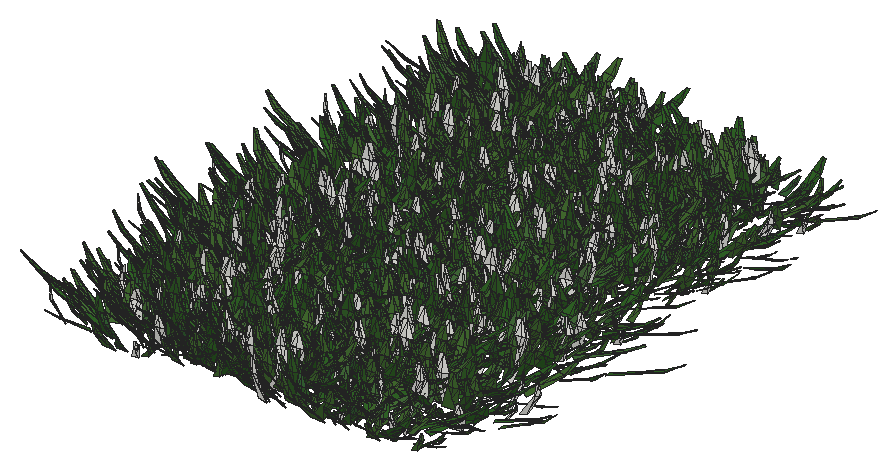
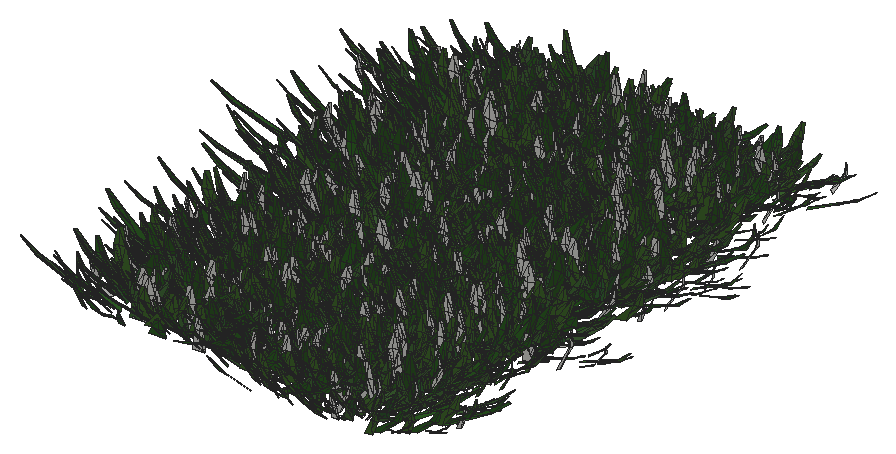
# SketchUp Ruby script. Lengths in inches.
U = 1.inch
M = Sketchup.active_model
def pt(a) = Geom::Point3d.new(a.map { |v| v * U })
def face(e, loops, mat)
  f = e.add_face(loops[0].map { |a| pt(a) })
  loops[1..].each { |l| e.add_face(l.map { |a| pt(a) }).erase! }
  f.material = f.back_material = mat if mat
  f
end
# faces: each face lists its corners as indices into pts; further lists are holes
def faces(e, pts, list, mat = nil) = list.each { |f| face(e, (f[0].is_a?(Array) ? f : [f]).map { |l| l.map { |i| pts[i] } }, mat) }
# xy, xz, yz: faces in a plane at the given z, y or x. An outline is a flat list of corners, or four numbers for a rectangle; further outlines are holes
def ring(l) = l.size == 4 ? [[l[0], l[1]], [l[2], l[1]], [l[2], l[3]], [l[0], l[3]]] : l.each_slice(2).to_a
def flat(e, list, mat, &to3) = list.each { |f| face(e, (f[0].is_a?(Array) ? f : [f]).map { |l| ring(l).map { |u, v| to3.(u, v) } }, mat) }
def xy(e, z, list, mat = nil) = flat(e, list, mat) { |x, y| [x, y, z] }
def xz(e, y, list, mat = nil) = flat(e, list, mat) { |x, z| [x, y, z] }
def yz(e, x, list, mat = nil) = flat(e, list, mat) { |y, z| [x, y, z] }
def lines(e, pts, list) = list.each { |a, b| e.add_line(pt(pts[a]), pt(pts[b])) }
# prism: a flat outline (further loops are holes) pulled along v
def prism(e, loops, v, mat = nil)
  f = face(e, loops, mat); d = Geom::Vector3d.new(v.map { |x| x * U })
  f.pushpull(f.normal.samedirection?(d) ? d.length : -d.length)
end
def box(e, o, s, mat = nil) = prism(e, [[o, [o[0] + s[0], o[1], o[2]], [o[0] + s[0], o[1] + s[1], o[2]], [o[0], o[1] + s[1], o[2]]]], [0, 0, s[2]], mat)
def at(x, y, z, deg = 0) = Geom::Transformation.translation(pt([x, y, z])) * Geom::Transformation.rotation(ORIGIN, Z_AXIS, deg.degrees)
def axes(o, x, y, z) = Geom::Transformation.new([*x, 0, *y, 0, *z, 0, *pt(o).to_a, 1])
def part(name) = M.definitions.add(name)
# library, detail: a bought-in or finely detailed component or shape, given as its bounding box
def library(name, o, s) = part(name).tap { |d| box(d.entities, o, s) }
def detail(e, o, s) = box(e.add_group.entities, o, s)
def put(e, d, t, mat = nil) = e.add_instance(d, t).tap { |i| i.material = mat if mat }
def group(e, t, mat = nil) = e.add_group.tap { |g| g.transformation = t; g.material = mat if mat }.entities
root = M.entities
M.materials.add("Material82").color = [68, 110, 58]
M.materials.add("Material83").color = [48, 90, 38]
M.materials.add("Material84").color = [68, 110, 48]
M.materials.add("Material85").color = [48, 90, 48]
M.materials.add("Material86").color = [58, 110, 58]
M.materials.add("Material87").color = [58, 90, 38]
M.materials.add("Material88").color = [68, 100, 58]
M.materials.add("Material89").color = [48, 100, 38]
c1 = part("grass00")
p = [[-0.6875,0.15,0],[-0.56,0.08,5.52],[-0.04,0.03,2.76],[0.48,-0.02,0],[0.35,-0.02,5.52],[-0.1,-0.14,5.52],
  [-0.12,0.65,8.37],[-0.42,0.65,8.37]]
faces(c1.entities,p,[[0,1,2,3],[3,2,4],[1,5,2],[5,4,2],[1,6,5],[4,5,6],[7,6,1]])
c2 = part("Group16\#1")
put(c2.entities,c1,axes([1.44,-0.61,-0.01],[0.05352,0.12609,0],[-0.10704,0.04543,0.07239],[0.06664,-0.02828,0.11628]),"Material85")
put(c2.entities,c1,axes([0.76,-0.15,-0.01],[0.04676,0.24062,0],[-0.23162,0.04501,0.06642],[0.0652,-0.01267,0.23595]),"Material82")
put(c2.entities,c1,axes([0.79,0.01,-0.01],[-0.00606,0.34651,0],[-0.34381,-0.00602,0.0432],[0.04319,0.00076,0.34386]))
put(c2.entities,c1,axes([1,0.23,-0.01],[-0.07192,0.31144,0],[-0.28722,-0.06632,0.1236],[0.12043,0.02781,0.29478]),"Material84")
put(c2.entities,c1,axes([1.66,0.77,-0.01],[-0.13828,0.29651,0],[-0.21551,-0.1005,0.22471],[0.20365,0.09498,0.23779]),"Material89")
put(c2.entities,c1,axes([0.6875,0.52,-0.01],[-0.18126,0.24051,0],[-0.22746,-0.17142,0.09788],[0.07817,0.05891,0.28481]),"Material84")
put(c2.entities,c1,axes([0.68,0.78,-0.01],[-0.215,0.18688,0],[-0.12385,-0.14248,0.21334],[0.13995,0.16101,0.18878]),"Material82")
put(c2.entities,c1,axes([0.56,1,-0.01],[-0.13756,0.07624,0],[-0.06159,-0.11112,0.0927],[0.04494,0.08108,0.12705]),"Material84")
put(c2.entities,c1,axes([0.2,0.64,-0.01],[-0.23729,0.07254,0],[-0.05711,-0.18681,0.153],[0.04473,0.14632,0.19535]),"Material89")
put(c2.entities,c1,axes([0.0625,0.72,-0.01],[-0.28874,0.02525,0],[-0.02179,-0.24916,0.14647],[0.01276,0.14591,0.25012]),"Material82")
put(c2.entities,c1,axes([-0.08,0.62,-0.01],[-0.34089,-0.04187,0],[0.03255,-0.26504,0.216],[-0.02633,0.21439,0.26703]),"Material89")
put(c2.entities,c1,axes([-0.34,0.98,-0.01],[-0.14314,-0.0493,0],[0.04397,-0.12769,0.06843],[-0.02228,0.0647,0.13505]),"Material89")
put(c2.entities,c1,axes([-0.87,1.45,-0.01],[-0.23488,-0.14114,0],[0.13761,-0.22901,0.06087],[-0.03135,0.05217,0.26717]))
put(c2.entities,c1,axes([-0.72,0.77,-0.01],[-0.14208,-0.13251,0],[0.07209,-0.0773,0.16301],[-0.11118,0.11922,0.1057]),"Material89")
put(c2.entities,c1,axes([-0.62,0.43,-0.01],[-0.14845,-0.21203,0],[0.18654,-0.13061,0.12304],[-0.10079,0.07057,0.22772]),"Material82")
put(c2.entities,c1,axes([-0.68,0.29,-0.01],[-0.13639,-0.32136,0],[0.31723,-0.13464,0.05579],[-0.05136,0.0218,0.34462]),"Material83")
put(c2.entities,c1,axes([-0.64,0.125,-0.01],[-0.0458,-0.23569,0],[0.22124,-0.043,0.08276],[-0.08124,0.01579,0.22538]),"Material86")
put(c2.entities,c1,axes([-1.6,-0.03,-0.01],[0.00576,-0.32897,0],[0.27526,0.00482,0.18018],[-0.18015,-0.00315,0.2753]),"Material84")
put(c2.entities,c1,axes([-1.36,-0.31,-0.01],[0.05718,-0.24765,0],[0.18172,0.04196,0.17267],[-0.16825,-0.03885,0.1865]),"Material89")
put(c2.entities,c1,axes([-1.54,-0.72,-0.01],[0.06537,-0.14017,0],[0.13555,0.06321,0.03939],[-0.0357,-0.01665,0.14956]))
put(c2.entities,c1,axes([-1.19,-0.9,-0.01],[0.09597,-0.12735,0],[0.11214,0.08451,0.07557],[-0.06035,-0.04548,0.14042]),"Material88")
put(c2.entities,c1,axes([-0.47,-0.54,-0.01],[0.11588,-0.10072,0],[0.0618,0.0711,0.12124],[-0.07953,-0.0915,0.0942]))
put(c2.entities,c1,axes([-0.47,-0.84,-0.01],[0.11927,-0.0661,0],[0.06603,0.11913,0.00646],[-0.00313,-0.00565,0.13621]),"Material84")
put(c2.entities,c1,axes([-0.38,-1.24,-0.01],[0.28037,-0.08571,0],[0.0618,0.20215,0.20315],[-0.05939,-0.19428,0.21139]),"Material88")
put(c2.entities,c1,axes([-0.06,-0.66,-0.01],[0.22719,-0.01987,0],[0.01247,0.14255,0.17758],[-0.01547,-0.17691,0.1431]),"Material87")
put(c2.entities,c1,axes([0.11,-0.89,-0.01],[0.14882,0.01828,0],[-0.01058,0.08611,0.12229],[0.01491,-0.12138,0.08676]),"Material85")
put(c2.entities,c1,axes([0.25,-0.72,-0.01],[0.20481,0.07053,0],[-0.06206,0.18022,0.10291],[0.03351,-0.0973,0.1906]),"Material85")
put(c2.entities,c1,axes([0.85,-1.42,-0.01],[0.16481,0.09904,0],[-0.09472,0.15762,0.05616],[0.02893,-0.04814,0.18389]),"Material84")
put(c2.entities,c1,axes([1.01,-1.09,-0.01],[0.21858,0.20385,0],[-0.17495,0.1876,0.15339],[0.10462,-0.11218,0.25652]),"Material89")
put(c2.entities,c1,axes([1.01,-0.71,-0.01],[0.08733,0.12473,0],[-0.06445,0.04512,0.13037],[0.1068,-0.07477,0.07867]),"Material85")
c3 = part("Group15\#1")
put(c3.entities,c2,at(0,0,0))
c4 = part("3darcstudiotree_grass00\#1")
put(c4.entities,c3,at(0,0,0))
put(root,c4,axes([1703.49,1033.95,-29.74],[4.10302,-0.30694,0],[0.8385,1.74326,-0.00778],[0.00611,0.0127,1.42033]))
put(root,c4,axes([1703.88,1017.02,-29.74],[-2.0309,1.41107,0],[-3.96455,-0.88745,-0.03094],[-0.10652,-0.02384,1.35284]))
put(root,c4,axes([1703.7,1018.32,-29.74],[3.97679,-0.10087,0],[0.2922,1.7917,-0.04097],[0.01281,0.07857,1.66267]))
put(root,c4,axes([1704.37,1024.5,-29.74],[2.96266,-0.9536,0],[2.21709,1.07131,-0.03627],[0.16479,0.07963,1.88825]))
put(root,c4,axes([1705.53,1009.61,-29.74],[-2.64678,-1.36079,0],[3.05956,-0.92555,-0.03114],[0.16031,-0.04849,1.87535]))
put(root,c4,axes([1704.94,1048.64,-29.74],[2.77032,-1.11765,0],[2.79461,1.07735,-0.00015],[0.00071,0.00027,1.98495]))
put(root,c4,axes([1704.06,1012.55,-29.74],[1.36747,1.27936,0],[-3.91602,0.651,-0.04214],[-0.23603,0.03924,1.93625]))
put(root,c4,axes([1705.93,1031.41,-29.74],[-0.46652,-1.63259,0],[3.80254,-0.169,-0.02839],[0.12966,-0.00576,1.31807]))
put(root,c4,axes([1706.04,1038.09,-29.74],[-2.24585,-1.17679,0],[2.75058,-0.81643,-0.02546],[0.1532,-0.04547,1.94365]))
put(root,c4,axes([1706.63,1047.5,-29.74],[-3.1613,-1.38915,0],[3.20855,-1.13563,-0.02493],[0.08224,-0.02911,1.43253]))
put(root,c4,axes([1706.375,1051.55,-29.74],[-4.11217,-0.39094,0],[0.86082,-1.40827,-0.01967],[0.02693,-0.04406,1.60841]))
put(root,c4,axes([1705.74,1021.11,-29.74],[-2.52022,1.35688,0],[-2.71694,-0.78485,-0.02032],[-0.10759,-0.03108,1.65635]))
put(root,c4,axes([1706.38,1001.24,-29.74],[-3.93546,0.24929,0],[-0.63824,-1.56709,-0.04907],[-0.04216,-0.10352,1.63442]))
put(root,c4,axes([1705.97,1040.7,-29.74],[1.48309,-1.18944,0],[3.17184,0.61511,-0.04022],[0.27217,0.05278,1.99791]))
put(root,c4,axes([1705.13,998.44,-29.74],[-0.1961,1.67231,0],[-3.9427,-0.07191,-0.00948],[-0.04368,-0.0008,1.36423]))
put(root,c4,axes([1706.89,1042.42,-29.74],[-1.75334,-1.53625,0],[3.78301,-0.67151,-0.04331],[0.23983,-0.04257,1.88835]))
put(root,c4,axes([1707.03,1045.07,-29.74],[-1.47837,-1.71881,0],[3.4357,-0.4596,-0.01224],[0.08437,-0.01129,1.97883]))
put(root,c4,axes([1705.26,1022.94,-29.74],[0.89151,1.73156,0],[-4.53511,0.36315,-0.02679],[-0.1364,0.01092,1.80175]))
put(root,c4,axes([1705.84,1002.9,-29.74],[3.29656,-0.16392,0],[0.52833,1.6525,-0.05027],[0.03097,0.09687,1.55905]))
put(root,c4,axes([1705.26,1035.78,-29.74],[1.8424,1.14237,0],[-3.65624,0.91712,-0.00074],[-0.00371,0.00093,1.93092]))
put(root,c4,axes([1706.68,1014.64,-29.74],[2.92684,-0.73502,0],[1.91435,1.18558,-0.0345],[0.12831,0.07947,1.8497]))
put(root,c4,axes([1706.88,1005.96,-29.74],[0.10092,1.39888,0],[-4.08431,0.04583,-0.02239],[-0.13434,0.00151,1.83839]))
put(root,c4,axes([1706.96,1029.15,-29.74],[-0.46714,1.44095,0],[-4.49775,-0.22678,-0.0277],[-0.15196,-0.00766,1.87956]))
put(root,c4,axes([1708.99,1019.2,-29.74],[-2.63576,-1.28026,0],[3.53005,-1.13032,-0.02494],[0.11128,-0.03563,1.95866]))
put(root,c4,axes([1708.95,1053.33,-29.74],[-3.99047,-0.40873,0],[1.06863,-1.62266,-0.00758],[0.01027,-0.0156,1.7185]))
put(root,c4,axes([1708.68,1029.42,-29.74],[-0.06008,-1.38054,0],[4.09358,-0.02771,-0.0405],[0.24938,-0.00169,1.89003]))
put(root,c4,axes([1709.07,1036.51,-29.74],[-1.38876,-1.54798,0],[3.56891,-0.49797,-0.03351],[0.18812,-0.02625,1.68972]))
put(root,c4,axes([1709.6875,1046.76,-29.74],[-0.94917,-1.78727,0],[4.28932,-0.35429,-0.02019],[0.10216,-0.00844,1.69814]))
put(root,c4,axes([1709.52,1052.08,-29.74],[-0.90047,-1.75818,0],[4.05941,-0.32336,-0.03802],[0.21461,-0.0171,1.78771]))
put(root,c4,axes([1709.85,1021.48,-29.74],[-2.86404,-0.64452,0],[1.81455,-1.25407,-0.04344],[0.15373,-0.10625,1.9596]))
put(root,c4,axes([1710.09,1009.37,-29.74],[-1.66133,-1.5225,0],[4.09169,-0.6944,-0.04688],[0.21591,-0.03664,1.67419]))
put(root,c4,axes([1710.02,1015.88,-29.74],[-3.61877,0.99301,0],[-2.17277,-1.23149,-0.01001],[-0.02667,-0.01512,1.32974]))
put(root,c4,axes([1711.03,1027.38,-29.74],[-0.34586,-1.45501,0],[4.09876,-0.15153,-0.00863],[0.04038,-0.00149,1.44957]))
put(root,c4,axes([1711.61,1014.23,-29.74],[-1.55676,-1.64059,0],[4.33421,-0.63965,-0.05081],[0.20494,-0.03024,1.49393]))
put(root,c4,axes([1710.2,1024.86,-29.74],[4.37611,-0.60729,0],[1.31361,1.47222,-0.0057],[0.0109,0.01221,1.70987]))
put(root,c4,axes([1711.69,1042.79,-29.74],[-0.47275,-1.4969,0],[4.46074,-0.21911,-0.06365],[0.35527,-0.01745,1.89522]))
put(root,c4,axes([1711.28,1038.82,-29.74],[2.20658,-1.37183,0],[2.86337,0.71632,-0.01781],[0.08885,0.02223,1.50117]))
put(root,c4,axes([1710.93,1049.89,-29.74],[3.60935,-0.56815,0],[1.37625,1.35979,-0.02611],[0.05001,0.04941,1.43783]))
put(root,c4,axes([1712.11,1002.8,-29.74],[-3.927,-0.17218,0],[0.45946,-1.62986,-0.05312],[0.03146,-0.11159,1.67036]))
put(root,c4,axes([1711.02,1000.79,-29.74],[4.2823,-0.66393,0],[1.32307,1.32724,-0.00849],[0.02062,0.02068,1.79934]))
put(root,c4,axes([1712.3,1033.72,-29.74],[0.52677,-1.54843,0],[3.37532,0.17859,-0.00096],[0.0064,0.00034,1.71349]))
put(root,c4,axes([1712.28,1031.74,-29.74],[-3.78642,0.03695,0],[-0.11198,-1.78455,-0.01248],[-0.00125,-0.01991,1.37214]))
put(root,c4,axes([1712.5,1045.21,-29.74],[-3.50363,0.54877,0],[-1.37004,-1.36042,-0.04199],[-0.09387,-0.09321,1.68502]))
put(root,c4,axes([1712.33,1023.08,-29.74],[-3.78815,1.05417,0],[-2.08305,-1.1642,0],[-0.00001,-0.00001,1.91868]))
put(root,c4,axes([1711.59,999.37,-29.74],[3.14187,0.39177,0],[-1.17778,1.46906,-0.04459],[-0.07661,0.09555,1.66873]))
put(root,c4,axes([1712.79,1040.2,-29.74],[-4.05008,0.95977,0],[-1.76425,-1.15789,-0.02116],[-0.06339,-0.0416,1.49339]))
put(root,c4,axes([1712.49,1005.88,-29.74],[-2.14427,1.00131,0],[-3.09998,-1.03248,-0.03207],[-0.1604,-0.05342,1.99077]))
put(root,c4,axes([1712.68,1007.9,-29.74],[-3.03453,1.36043,0],[-3.50876,-1.21725,-0.06393],[-0.1925,-0.06678,1.40472]))
put(root,c4,axes([1712.5,1011.48,-29.74],[4.55933,-0.17295,0],[0.45061,1.84755,-0.06081],[0.02387,0.09789,1.44654]))
put(root,c4,axes([1714.37,1026.73,-29.74],[-0.03672,-1.35909,0],[4.67682,-0.01965,-0.05216],[0.20276,-0.00085,1.36288]))
put(root,c4,axes([1714.47,1012.2,-29.74],[0.13892,-1.80916,0],[4.0915,0.04886,-0.01983],[0.09749,0.00116,1.50947]))
put(root,c4,axes([1714.72,1045.11,-29.74],[-0.70107,-1.67232,0],[4.13597,-0.26967,-0.0168],[0.0818,-0.00533,1.55067]))
put(root,c4,axes([1714.86,1016.1875,-29.74],[-3.75519,-1.14447,0],[2.68213,-1.36874,-0.06061],[0.1619,-0.08262,1.43628]))
put(root,c4,axes([1714.39,1028.91,-29.74],[-0.54027,-1.6401,0],[3.32557,-0.17038,-0.04034],[0.23473,-0.01203,1.47504]))
put(root,c4,axes([1714.625,1024.72,-29.74],[-3.58356,0.46021,0],[-1.0679,-1.2933,-0.04555],[-0.08783,-0.10637,1.60995]))
put(root,c4,axes([1715.09,1002.92,-29.74],[-3.8661,0.57248,0],[-1.34665,-1.41442,-0.01194],[-0.02505,-0.02631,1.71307]))
put(root,c4,axes([1715.29,1010.36,-29.74],[-3.59396,1.08002,0],[-2.30452,-1.19271,-0.04347],[-0.15376,-0.07958,1.66314]))
put(root,c4,axes([1716.07,999.57,-29.74],[-3.24117,-0.71309,0],[1.62667,-1.14993,-0.00653],[0.01841,-0.01301,1.4475]))
put(root,c4,axes([1716.42,1043.23,-29.74],[-3.07387,-1.37226,0],[2.57369,-0.89663,-0.00245],[0.01347,-0.00469,1.8862]))
put(root,c4,axes([1714.6875,1049.15,-29.74],[0.39811,1.50692,0],[-3.94981,0.16229,-0.02993],[-0.16157,0.00664,1.61572]))
put(root,c4,axes([1714.78,1022.58,-29.74],[-0.46786,1.28327,0],[-3.81344,-0.21623,-0.00494],[-0.02392,-0.00136,1.4129]))
put(root,c4,axes([1716.57,1005.55,-29.74],[0.52643,-1.67667,0],[4.29673,0.20982,-0.00236],[0.01155,0.00056,1.5989]))
put(root,c4,axes([1715.29,1046.66,-29.74],[3.86987,-0.34459,0],[0.79622,1.39073,-0.03599],[0.03867,0.06754,1.32194]))
put(root,c4,axes([1716.37,1031.85,-29.74],[-3.89357,0.61481,0],[-1.50479,-1.48217,-0.00598],[-0.01246,-0.01228,1.70205]))
put(root,c4,axes([1715.52,1007.16,-29.74],[4.26757,-0.1267,0],[0.26808,1.40432,-0.02417],[0.01226,0.06424,1.80918]))
put(root,c4,axes([1715.57,1050.8125,-29.74],[0.18137,1.61713,0],[-3.86456,0.06741,-0.03464],[-0.18684,0.00326,1.56527]))
put(root,c4,axes([1715.35,1052.95,-29.74],[2.68425,0.98126,0],[-3.08103,1.31083,-0.0132],[-0.04194,0.01784,1.58767]))
put(root,c4,axes([1717.13,1018.3,-29.74],[-4.03193,0.12785,0],[-0.33897,-1.66251,-0.04274],[-0.01416,-0.06944,1.31001]))
put(root,c4,axes([1717.47,1033.54,-29.74],[-2.54975,-1.13663,0],[2.74994,-0.95943,-0.02762],[0.1264,-0.0441,1.68176]))
put(root,c4,axes([1715.75,1020.33,-29.74],[2.51292,1.08795,0],[-3.26468,1.1728,-0.05824],[-0.20485,0.07359,1.57486]))
put(root,c4,axes([1716.92,1037.86,-29.74],[2.12492,-1.52639,0],[3.32667,0.72027,-0.02765],[0.13101,0.02837,1.53783]))
put(root,c4,axes([1716.25,1001.04,-29.74],[2.57949,0.81299,0],[-2.19489,1.0831,-0.04441],[-0.18645,0.09201,1.772]))
put(root,c4,axes([1717.17,1040.1,-29.74],[2.26224,-1.2031,0],[3.43735,1.00525,-0.03781],[0.13632,0.03987,1.4396]))
put(root,c4,axes([1716.34,1035.7,-29.74],[0.64746,1.71828,0],[-3.59,0.21039,-0.03328],[-0.18561,0.01088,1.53387]))
put(root,c4,axes([1717.41,1013.91,-29.74],[1.65411,1.32331,0],[-4.02119,0.78176,-0.01549],[-0.05875,0.01142,1.42146]))
put(root,c4,axes([1720.15,1000.57,-29.74],[-1.99996,-1.21087,0],[3.64955,-0.93751,-0.00487],[0.02184,-0.00561,1.74651]))
put(root,c4,axes([1719.93,1049.92,-29.74],[-4.08637,0.5893,0],[-1.1512,-1.24155,-0.04181],[-0.0785,-0.08466,1.37365]))
put(root,c4,axes([1720.2,1033.33,-29.74],[0.94723,-1.59052,0],[4.2139,0.39031,-0.04288],[0.2193,0.02031,1.70449]))
put(root,c4,axes([1720.4,1003.34,-29.74],[0.76825,-1.34447,0],[4.07723,0.36235,-0.02216],[0.10533,0.00936,1.52603]))
put(root,c4,axes([1721.03,1039.85,-29.74],[-4.28344,0.1007,0],[-0.25434,-1.68266,-0.00226],[-0.00079,-0.00521,1.87745]))
put(root,c4,axes([1720.7,1044.92,-29.74],[1.6756,-1.36696,0],[3.5262,0.67226,-0.03335],[0.16368,0.0312,1.60043]))
put(root,c4,axes([1721.32,1012.25,-29.74],[-0.47602,-1.5827,0],[4.1601,-0.1946,-0.02638],[0.12052,-0.00564,1.44452]))
put(root,c4,axes([1720.36,1036.29,-29.74],[4.15464,-0.59094,0],[1.53872,1.68251,-0.06016],[0.09162,0.10018,1.52593]))
put(root,c4,axes([1720.62,1020.84,-29.74],[-1.67139,1.30839,0],[-3.46219,-0.68786,-0.03585],[-0.17478,-0.03472,1.58646]))
put(root,c4,axes([1721.21,1027.42,-29.74],[-3.50073,0.942,0],[-2.16331,-1.25037,-0.04776],[-0.1565,-0.09046,1.6727]))
put(root,c4,axes([1720.56,1019.13,-29.74],[3.80678,-0.63656,0],[1.53404,1.42681,-0.02583],[0.05775,0.05372,1.68703]))
put(root,c4,axes([1720.96,1047.1875,-29.74],[4.59121,-0.45029,0],[0.84969,1.34743,-0.00031],[0.00049,0.00078,1.72722]))
put(root,c4,axes([1721.51,1013.65,-29.74],[3.46257,-0.87441,0],[2.25752,1.39035,-0.00312],[0.00811,0.00499,1.51309]))
put(root,c4,axes([1721.13,1016.7,-29.74],[4.45522,-0.42871,0],[0.88291,1.42703,-0.01844],[0.02851,0.04608,1.82062]))
put(root,c4,axes([1722.08,1038.17,-29.74],[2.11135,-1.17998,0],[3.12805,0.87051,-0.01427],[0.05324,0.01482,1.30992]))
put(root,c4,axes([1722.18,1007.3125,-29.74],[2.70908,-1.29001,0],[3.26836,1.0675,-0.01649],[0.07179,0.02345,1.79785]))
put(root,c4,axes([1722.91,1030.05,-29.74],[-1.99014,-1.36063,0],[3.61455,-0.82226,-0.05686],[0.20653,-0.04698,1.31145]))
put(root,c4,axes([1722.89,1051.25,-29.74],[-4.63629,0.17249,0],[-0.31305,-1.3087,-0.02738],[-0.01684,-0.0704,1.63584]))
put(root,c4,axes([1722.57,1025.35,-29.74],[1.2093,-1.57862,0],[4.10109,0.48862,-0.03916],[0.21176,0.02523,1.81408]))
put(root,c4,axes([1721.11,1031.42,-29.74],[2.22707,1.32751,0],[-3.83725,1.00121,-0.02773],[-0.10131,0.02643,1.51065]))
put(root,c4,axes([1721.9,1042.79,-29.74],[0.32393,1.2922,0],[-3.8703,0.1509,-0.01511],[-0.10076,0.00393,1.95375]))
put(root,c4,axes([1722.09,1004.77,-29.74],[3.29328,0.79365,0],[-2.38723,1.54066,-0.04231],[-0.12354,0.07973,1.92144]))
put(root,c4,axes([1723.81,1010.29,-29.74],[-4.33123,0.18779,0],[-0.372,-1.33439,-0.04038],[-0.02759,-0.09898,1.5952]))
put(root,c4,axes([1723.45,999.125,-29.74],[-2.43738,1.19248,0],[-2.72185,-0.86527,-0.02131],[-0.12,-0.03815,1.8955]))
put(root,c4,axes([1723.4,1023.49,-29.74],[-1.08989,1.28976,0],[-3.11811,-0.40981,-0.02384],[-0.1661,-0.02183,1.80943]))
put(root,c4,axes([1725.3,1031.61,-29.74],[0.31301,-1.31124,0],[3.5948,0.13346,-0.01523],[0.11152,0.00414,1.99019]))
put(root,c4,axes([1725.86,1004.77,-29.74],[-3.40339,-1.11564,0],[2.13204,-1.01156,-0.01701],[0.08509,-0.04037,1.95649]))
put(root,c4,axes([1726.22,1017.9,-29.74],[-3.55731,-0.39699,0],[0.91028,-1.26863,-0.03071],[0.04629,-0.06451,1.38702]))
put(root,c4,axes([1725.72,1012.59,-29.74],[1.53941,-1.17663,0],[3.76142,0.76538,-0.04957],[0.23972,0.04878,1.72633]))
put(root,c4,axes([1726.2,1043.03,-29.74],[-0.12409,-1.44715,0],[3.33282,-0.04445,-0.02047],[0.13634,-0.00182,1.66543]))
put(root,c4,axes([1725.92,1010.14,-29.74],[1.91221,-1.68967,0],[4.00415,0.70478,-0.04062],[0.20203,0.03556,1.79015]))
put(root,c4,axes([1725.85,1040.36,-29.74],[-2.75564,1.16599,0],[-3.11928,-1.14656,-0.00031],[-0.00116,-0.00043,1.61707]))
put(root,c4,axes([1725.78,1016.95,-29.74],[3.14616,-0.46124,0],[1.36147,1.44435,-0.02775],[0.06352,0.06739,1.92398]))
put(root,c4,axes([1727.18,1025.6,-29.74],[-0.59398,-1.49967,0],[3.68059,-0.22673,-0.04759],[0.22724,-0.014,1.34947]))
put(root,c4,axes([1727.74,1038.39,-29.74],[-1.90322,-1.23489,0],[2.93996,-0.70472,-0.04312],[0.27444,-0.06578,1.92045]))
put(root,c4,axes([1727.91,1047.59,-29.74],[-2.12705,-1.09895,0],[2.82257,-0.84968,-0.04177],[0.17079,-0.05141,1.36919]))
put(root,c4,axes([1728.03,1014.16,-29.74],[1.44153,-1.60776,0],[3.23959,0.45176,-0.02361],[0.11408,0.01591,1.32009]))
put(root,c4,axes([1727.07,1045.27,-29.74],[1.45904,1.69634,0],[-4.12454,0.55175,-0.04327],[-0.22093,0.02955,1.7601]))
put(root,c4,axes([1727.26,1033.61,-29.74],[0.41076,1.77313,0],[-3.60416,0.12986,-0.02215],[-0.11578,0.00417,1.42375]))
put(root,c4,axes([1728.44,1036.79,-29.74],[0.96466,-1.81909,0],[3.32191,0.27398,-0.01603],[0.09156,0.00755,1.48463]))
put(root,c4,axes([1727.46,1008.52,-29.74],[-0.86085,1.83609,0],[-4.61027,-0.33618,-0.00297],[-0.01572,-0.00115,1.8915]))
put(root,c4,axes([1727.75,1050.66,-29.74],[3.95759,-0.11816,0],[0.2883,1.50178,-0.04662],[0.02067,0.10765,1.68074]))
put(root,c4,axes([1727.9,1049.83,-29.74],[-0.65253,1.4678,0],[-3.82967,-0.26479,-0.02601],[-0.14603,-0.0101,1.66111]))
put(root,c4,axes([1727.38,1001.16,-29.74],[2.91821,1.08875,0],[-2.82314,1.17688,-0.00432],[-0.01382,0.00576,1.43292]))
put(root,c4,axes([1728.64,1029.41,-29.74],[3.48292,-0.82099,0],[2.25154,1.48559,-0.05659],[0.14545,0.09597,1.64805]))
put(root,c4,axes([1728.09,998.86,-29.74],[4.39717,0.52423,0],[-1.00944,1.31686,-0.04581],[-0.07981,0.10411,1.57403]))
put(root,c4,axes([1728.07,1027.59,-29.74],[3.42406,1.01361,0],[-2.506,1.31662,-0.02233],[-0.08435,0.04432,1.9689]))
put(root,c4,axes([1728.78,1020.98,-29.74],[-2.64058,1.54622,0],[-3.55505,-0.94424,-0.0002],[-0.001,-0.00026,1.96126]))
put(root,c4,axes([1729.125,1022.34,-29.74],[4.33275,-0.34682,0],[0.77843,1.5125,-0.04034],[0.04996,0.09707,1.82611]))
put(root,c4,axes([1730.94,1047.06,-29.74],[-3.32048,-0.89448,0],[2.67505,-1.54445,-0.03279],[0.08824,-0.05095,1.69581]))
put(root,c4,axes([1729.09,1004.125,-29.74],[3.65442,0.79234,0],[-1.92667,1.38205,-0.0244],[-0.05154,0.03697,1.31386]))
put(root,c4,axes([1731.51,1023.16,-29.74],[-4.47242,-0.43212,0],[1.12449,-1.81009,-0.038],[0.04833,-0.0778,1.89315]))
put(root,c4,axes([1731.48,1040.74,-29.74],[3.41982,0.22152,0],[-0.58321,1.40029,-0.00501],[-0.00425,0.0102,1.40942]))
put(root,c4,axes([1731.42,1050.02,-29.74],[0.62564,1.8219,0],[-4.46763,0.23861,-0.03426],[-0.17796,0.0095,1.77113]))
put(root,c4,axes([1732.125,1034.15,-29.74],[3.06207,-0.55792,0],[1.42852,1.21938,-0.0238],[0.07482,0.06387,1.9133]))
put(root,c4,axes([1732.59,1016.52,-29.74],[2.42149,-1.19086,0],[3.28427,1.03866,-0.04277],[0.16953,0.05361,1.60323]))
put(root,c4,axes([1733.55,1005.76,-29.74],[-4.5051,-0.1347,0],[0.33952,-1.76605,-0.05601],[0.0175,-0.09103,1.39118]))
put(root,c4,axes([1733.68,1009.92,-29.74],[-3.05686,-1.19982,0],[3.00062,-1.189,-0.05331],[0.20258,-0.08027,1.71744]))
put(root,c4,axes([1733.67,1007.22,-29.74],[0.58993,-1.49665,0],[4.0908,0.25078,-0.01704],[0.09795,0.00601,1.80481]))
put(root,c4,axes([1732.22,1002.86,-29.74],[0.93986,1.81776,0],[-4.11362,0.3308,-0.03996],[-0.17618,0.01417,1.416]))
put(root,c4,axes([1732.23,1031.26,-29.74],[1.86,1.67689,0],[-3.22779,0.55683,-0.02724],[-0.14202,0.0245,1.50258]))
put(root,c4,axes([1732.51,1014.91,-29.74],[3.80375,0.01195,0],[-0.02861,1.41659,-0.01492],[-0.00081,0.04025,1.84219]))
put(root,c4,axes([1732.55,999.27,-29.74],[3.00521,0.63807,0],[-1.62064,1.18715,-0.02125],[-0.05194,0.03805,1.32121]))
put(root,c4,axes([1733.42,1050.73,-29.74],[-2.17573,1.65884,0],[-3.97455,-0.81077,-0.04288],[-0.19169,-0.0391,1.68813]))
put(root,c4,axes([1733.58,1025.03,-29.74],[-1.91722,1.31385,0],[-4.0358,-0.91594,-0.03664],[-0.12047,-0.02734,1.3241]))
put(root,c4,axes([1733.33,1038.56,-29.74],[2.76774,0.7917,0],[-1.93345,1.05126,-0.02439],[-0.09329,0.05072,1.60766]))
put(root,c4,axes([1733.82,1018.54,-29.74],[4.38931,-0.45982,0],[1.18067,1.75286,-0.06211],[0.07411,0.11002,1.60192]))
put(root,c4,axes([1734.59,1042.83,-29.74],[1.79387,-1.26785,0],[3.18419,0.70071,-0.05199],[0.23586,0.0519,1.41973]))
put(root,c4,axes([1734.27,1036.38,-29.74],[-1.97144,1.08801,0],[-3.33394,-0.93955,-0.01309],[-0.05439,-0.01533,1.56859]))
